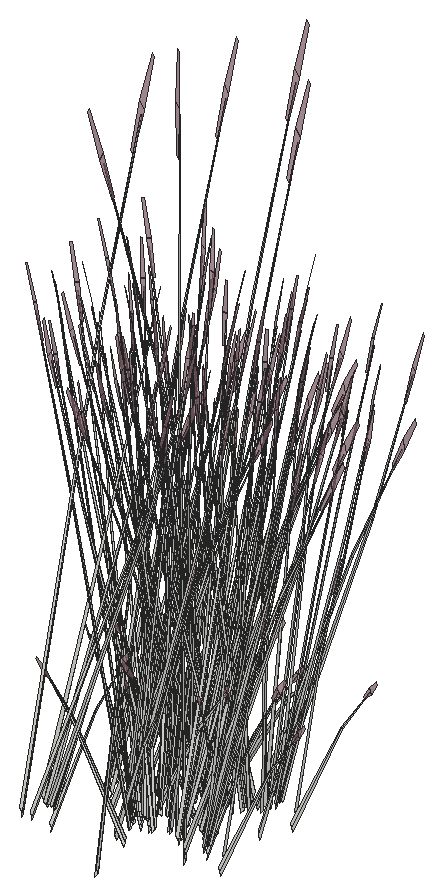
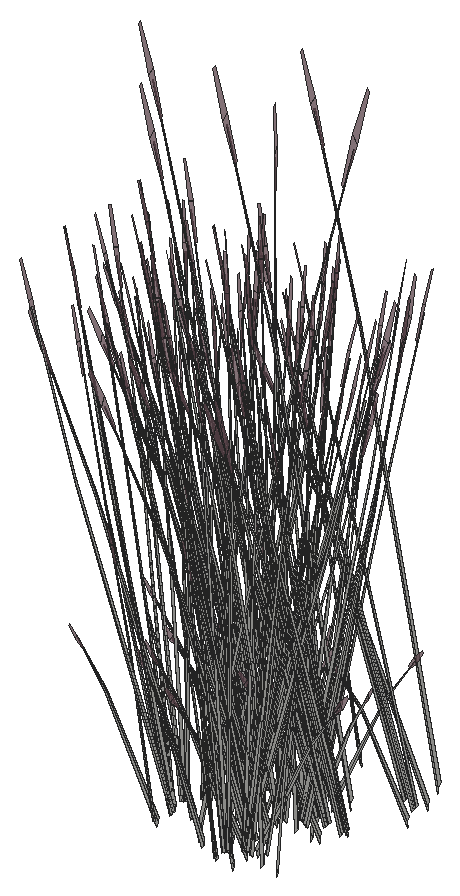
# SketchUp Ruby script. Lengths in inches.
U = 1.inch
M = Sketchup.active_model
def pt(a) = Geom::Point3d.new(a.map { |v| v * U })
def face(e, loops, mat)
  f = e.add_face(loops[0].map { |a| pt(a) })
  loops[1..].each { |l| e.add_face(l.map { |a| pt(a) }).erase! }
  f.material = f.back_material = mat if mat
  f
end
# faces: each face lists its corners as indices into pts; further lists are holes
def faces(e, pts, list, mat = nil) = list.each { |f| face(e, (f[0].is_a?(Array) ? f : [f]).map { |l| l.map { |i| pts[i] } }, mat) }
# xy, xz, yz: faces in a plane at the given z, y or x. An outline is a flat list of corners, or four numbers for a rectangle; further outlines are holes
def ring(l) = l.size == 4 ? [[l[0], l[1]], [l[2], l[1]], [l[2], l[3]], [l[0], l[3]]] : l.each_slice(2).to_a
def flat(e, list, mat, &to3) = list.each { |f| face(e, (f[0].is_a?(Array) ? f : [f]).map { |l| ring(l).map { |u, v| to3.(u, v) } }, mat) }
def xy(e, z, list, mat = nil) = flat(e, list, mat) { |x, y| [x, y, z] }
def xz(e, y, list, mat = nil) = flat(e, list, mat) { |x, z| [x, y, z] }
def yz(e, x, list, mat = nil) = flat(e, list, mat) { |y, z| [x, y, z] }
def lines(e, pts, list) = list.each { |a, b| e.add_line(pt(pts[a]), pt(pts[b])) }
# prism: a flat outline (further loops are holes) pulled along v
def prism(e, loops, v, mat = nil)
  f = face(e, loops, mat); d = Geom::Vector3d.new(v.map { |x| x * U })
  f.pushpull(f.normal.samedirection?(d) ? d.length : -d.length)
end
def box(e, o, s, mat = nil) = prism(e, [[o, [o[0] + s[0], o[1], o[2]], [o[0] + s[0], o[1] + s[1], o[2]], [o[0], o[1] + s[1], o[2]]]], [0, 0, s[2]], mat)
def at(x, y, z, deg = 0) = Geom::Transformation.translation(pt([x, y, z])) * Geom::Transformation.rotation(ORIGIN, Z_AXIS, deg.degrees)
def axes(o, x, y, z) = Geom::Transformation.new([*x, 0, *y, 0, *z, 0, *pt(o).to_a, 1])
def part(name) = M.definitions.add(name)
# library, detail: a bought-in or finely detailed component or shape, given as its bounding box
def library(name, o, s) = part(name).tap { |d| box(d.entities, o, s) }
def detail(e, o, s) = box(e.add_group.entities, o, s)
def put(e, d, t, mat = nil) = e.add_instance(d, t).tap { |i| i.material = mat if mat }
def group(e, t, mat = nil) = e.add_group.tap { |g| g.transformation = t; g.material = mat if mat }.entities
root = M.entities
M.materials.add("LightPink_Translucent").color = [144, 107, 117]
M.materials["LightPink_Translucent"].alpha = 0.75
c1 = part("blade")
p = [[2.15,0.21,22],[0,0.17,0],[0.09,0.45,0],[2.18,0.31,22],[2.29,0.31,22],[0.38,0.45,0],
  [2.48,0.24,33],[2.49,0.24,33],[2.48,0.22,33]]
faces(c1.entities,p,[[0,1,2,3],[4,5,2,3],[6,3,4,7],[8,0,3,6]])
c2 = part("seeds")
p = [[0.3,-0.1,1.38],[-0.01,-0.03,1.59],[-0.01,-0.03,0.03],[0.14,-0.07,-0.07],[0.29,-0.03,3],[0.15,0.01,3.11]]
faces(c2.entities,p,[[0,1,2,3],[1,0,4,5]],"LightPink_Translucent")
c3 = part("blade with seeds")
put(c3.entities,c1,at(0,0,0))
put(c3.entities,c2,axes([2.4,0.25,30.99],[1.5799,-0.05474,1.17369],[-0.12525,1.92788,0.29478],[-0.07173,-0.02425,1.56792]))
put(root,c3,axes([337.16,22.48,50.44],[0.32236,-0.02796,1.01491],[-0.20448,0.24636,0.74569],[-0.1593,-0.03696,0.22354]))
put(root,c3,axes([333,21.07,52.4],[0.50473,0.00941,-0.62776],[-0.0339,0.39618,0.07576],[0.21383,0.04181,0.88802]))
put(root,c3,axes([336.36,22.91,50.44],[-0.16818,0.19891,1.01491],[-0.14456,-0.26725,0.74569],[0.1389,-0.06697,0.22354]))
put(root,c3,axes([338.18,21.87,52.45],[-0.02704,0.39739,-0.10745],[-0.51189,-0.01086,-0.59638],[-0.19715,-0.0276,0.90619]))
put(root,c3,axes([342.01,23.39,52.45],[-0.25405,-0.35383,-0.10745],[0.45089,-0.17388,-0.59638],[0.19001,-0.04668,0.90619]))
put(root,c3,axes([341.98,23.09,52.14],[0.13679,-0.35544,-0.45151],[0.46898,0.12183,-0.34973],[0.18882,-0.03259,0.86392]))
put(root,c3,axes([338.31,18.42,50.97],[0.01109,-0.20172,1.3638],[0.49896,0.10655,0.18846],[-0.04323,0.21498,0.64398]))
put(root,c3,axes([336.12,23.66,52],[0.43951,-0.05584,-0.31292],[0.11606,0.31924,0.40398],[0.12595,-0.08575,0.77298]))
put(root,c3,axes([333.31,21.23,52],[0.28729,0.24465,-0.31292],[-0.32804,0.23159,0.40398],[0.16667,0.03524,0.77298]))
put(root,c3,axes([341.9,23.22,52.4],[0.44368,-0.17257,-0.62776],[0.24726,0.35524,0.07576],[0.21437,-0.04035,0.88802]))
put(root,c3,axes([332.28,20.6,51.43],[-0.18755,-0.06732,1.51428],[0.38813,-0.28243,0.12244],[0.24191,0.12741,0.64734]))
put(root,c3,axes([332.3125,19.72,51.95],[-0.4363,-0.20303,1.22187],[0.46069,-0.31611,0.5272],[0.14077,0.1905,1.18105]))
put(root,c3,axes([332.97,21.37,50.44],[-0.28429,-0.11236,1.01491],[0.36709,-0.11416,0.74569],[0.09901,0.0967,0.22354]))
put(root,c3,axes([342.27,23.25,52],[0.41962,0.10901,-0.31292],[-0.12239,0.31802,0.40398],[0.16894,-0.02916,0.77298]))
put(root,c3,axes([331.97,21.69,52.45],[0.30087,-0.33447,-0.10745],[0.43572,0.19269,-0.59638],[0.15146,0.0945,0.90619]))
put(root,c3,axes([341.13,22.86,51.43],[-0.20943,0.00885,1.51428],[0.13893,-0.38357,0.12244],[0.29846,0.02372,0.64734]))
put(root,c3,axes([332.33,21.52,52.14],[0.49824,-0.09289,-0.45151],[0.08716,0.35177,-0.34973],[0.13382,0.10081,0.86392]))
put(root,c3,axes([335.96,26.6,52.4],[-0.24099,-0.31773,-0.62776],[0.49607,-0.17707,0.07576],[-0.05635,-0.15352,0.88802]))
put(root,c3,axes([336.01,24.72,52.45],[-0.25405,-0.35383,-0.10745],[0.45089,-0.17388,-0.59638],[0.19001,-0.04668,0.90619]))
put(root,c3,axes([335.98,24.42,52.14],[0.13679,-0.35544,-0.45151],[0.46898,0.12183,-0.34973],[0.18882,-0.03259,0.86392]))
put(root,c3,axes([336.96,26.91,52.4],[0.01314,-0.36145,-0.62776],[0.55324,0.02428,0.07576],[0.05838,-0.15313,0.88802]))
put(root,c3,axes([335.9,24.55,52.4],[0.44368,-0.17257,-0.62776],[0.24726,0.35524,0.07576],[0.21437,-0.04035,0.88802]))
put(root,c3,axes([343.16,23.32,50.44],[-0.31197,0.06451,1.01491],[0.14684,-0.26661,0.74569],[0.1655,0.01824,0.22354]))
put(root,c3,axes([336,26.33,52],[0.15222,-0.30049,-0.31292],[0.44409,0.08764,0.40398],[-0.04072,-0.12098,0.77298]))
put(root,c3,axes([336.34,26.73,51.43],[-0.09401,0.13431,1.51428],[-0.3944,-0.27795,0.12244],[0.17792,-0.17323,0.64734]))
put(root,c3,axes([335.78,26.54,52.14],[-0.49634,-0.09796,-0.45151],[0.17013,-0.33585,-0.34973],[-0.04551,-0.13522,0.86392]))
put(root,c3,axes([336.08,25.7,50.44],[0.06477,0.22786,1.01491],[-0.35932,-0.1262,0.74569],[0.03867,-0.11667,0.22354]))
put(root,c3,axes([336.85,26.79,52.14],[-0.36145,-0.26255,-0.45151],[0.38183,-0.22994,-0.34973],[0.055,-0.1334,0.86392]))
put(root,c3,axes([337.63,22.91,52.14],[-0.13679,0.35544,-0.45151],[-0.46898,-0.12183,-0.34973],[-0.18882,0.03259,0.86392]))
put(root,c3,axes([337.61,22.6,52.45],[0.25405,0.35383,-0.10745],[-0.45089,0.17388,-0.59638],[-0.19001,0.04668,0.90619]))
put(root,c3,axes([342.62,24.14,51.47],[-0.09664,-0.32847,-0.03085],[0.45676,-0.07551,-0.13989],[0.09538,0.02082,0.4614]))
put(root,c3,axes([341.4375,24.13,52.45],[0.02704,-0.39739,-0.10745],[0.51189,0.01086,-0.59638],[0.19715,0.0276,0.90619]))
put(root,c3,axes([338.69,27.6,51.43],[0.11542,0.12546,1.51428],[-0.53333,0.10562,0.12244],[-0.12054,-0.19696,0.64734]))
put(root,c3,axes([336.2,26.52,52.45],[-0.49409,0.18193,-0.10745],[-0.24281,-0.32289,-0.59638],[-0.06519,-0.13607,0.90619]))
put(root,c3,axes([337.23,26.93,52.45],[-0.55492,-0.01936,-0.10745],[0.01517,-0.36657,-0.59638],[0.03855,-0.14118,0.90619]))
put(root,c3,axes([336.27,24.58,52],[0.41962,0.10901,-0.31292],[-0.12239,0.31802,0.40398],[0.16894,-0.02916,0.77298]))
put(root,c3,axes([337.19,26.69,52],[0.34164,-0.20573,-0.31292],[0.3234,0.23491,0.40398],[0.04921,-0.11936,0.77298]))
put(root,c3,axes([340.11,27.69,52.4],[-0.24099,-0.31773,-0.62776],[0.49607,-0.17707,0.07576],[-0.05635,-0.15352,0.88802]))
put(root,c3,axes([335.13,24.18,51.43],[-0.20943,0.00885,1.51428],[0.13893,-0.38357,0.12244],[0.29846,0.02372,0.64734]))
put(root,c3,axes([341.12,28.01,52.4],[0.01314,-0.36145,-0.62776],[0.55324,0.02428,0.07576],[0.05838,-0.15313,0.88802]))
put(root,c3,axes([341.46,23.9375,52.4],[0.50473,0.00941,-0.62776],[-0.0339,0.39618,0.07576],[0.21383,0.04181,0.88802]))
put(root,c3,axes([340.16,27.42,52],[0.15222,-0.30049,-0.31292],[0.44409,0.08764,0.40398],[-0.04072,-0.12098,0.77298]))
put(root,c3,axes([340.5,27.82,51.43],[-0.09401,0.13431,1.51428],[-0.3944,-0.27795,0.12244],[0.17792,-0.17323,0.64734]))
put(root,c3,axes([339.93,27.63,52.14],[-0.49634,-0.09796,-0.45151],[0.17013,-0.33585,-0.34973],[-0.04551,-0.13522,0.86392]))
put(root,c3,axes([340.24,26.79,50.44],[0.06477,0.22786,1.01491],[-0.35932,-0.1262,0.74569],[0.03867,-0.11667,0.22354]))
put(root,c3,axes([337.16,24.64,50.44],[-0.31197,0.06451,1.01491],[0.14684,-0.26661,0.74569],[0.1655,0.01824,0.22354]))
put(root,c3,axes([341.01,27.89,52.14],[-0.36145,-0.26255,-0.45151],[0.38183,-0.22994,-0.34973],[0.055,-0.1334,0.86392]))
put(root,c3,axes([337.61,27.54,52.4],[0.26374,-0.30832,-0.62776],[0.46217,0.21911,0.07576],[0.15748,-0.11171,0.88802]))
put(root,c3,axes([337.6,27.4,52.14],[-0.12971,-0.3568,-0.45151],[0.49122,-0.06241,-0.34973],[0.14077,-0.09583,0.86392]))
put(root,c3,axes([336.7,24.43,50.44],[0.21042,-0.1771,1.01491],[0.08303,0.28036,0.74569],[-0.15207,0.0502,0.22354]))
put(root,c3,axes([341.77,24.1,52],[0.28729,0.24465,-0.31292],[-0.32804,0.23159,0.40398],[0.16667,0.03524,0.77298]))
put(root,c3,axes([337.49,23.66,52],[-0.43951,0.05584,-0.31292],[-0.11606,-0.31924,0.40398],[-0.12595,0.08575,0.77298]))
put(root,c3,axes([337.83,27.65,52.45],[-0.46706,-0.21546,-0.10745],[0.26908,-0.31203,-0.59638],[0.13196,-0.10846,0.90619]))
put(root,c3,axes([340.36,27.61,52.45],[-0.49409,0.18193,-0.10745],[-0.24281,-0.32289,-0.59638],[-0.06519,-0.13607,0.90619]))
put(root,c3,axes([336.62,25.46,51.47],[-0.09664,-0.32847,-0.03085],[0.45676,-0.07551,-0.13989],[0.09538,0.02082,0.4614]))
put(root,c3,axes([341.38,28.02,52.45],[-0.55492,-0.01936,-0.10745],[0.01517,-0.36657,-0.59638],[0.03855,-0.14118,0.90619]))
put(root,c3,axes([341.35,27.79,52],[0.34164,-0.20573,-0.31292],[0.3234,0.23491,0.40398],[0.04921,-0.11936,0.77298]))
put(root,c3,axes([335.4375,25.45,52.45],[0.02704,-0.39739,-0.10745],[0.51189,0.01086,-0.59638],[0.19715,0.0276,0.90619]))
put(root,c3,axes([338.39,27.0625,50.44],[0.26338,0.136,1.01491],[-0.38358,0.08175,0.74569],[-0.08207,-0.10452,0.22354]))
put(root,c3,axes([339.03,27.78,52.4],[-0.43054,-0.18887,-0.62776],[0.30598,-0.33097,0.07576],[-0.15599,-0.11277,0.88802]))
put(root,c3,axes([338.88,27.53,52],[-0.07798,-0.31474,-0.31292],[0.44579,-0.08311,0.40398],[-0.11974,-0.09019,0.77298]))
put(root,c3,axes([340.73,23.47,51.43],[-0.18755,-0.06732,1.51428],[0.38813,-0.28243,0.12244],[0.24191,0.12741,0.64734]))
put(root,c3,axes([340.77,22.59,51.95],[-0.4363,-0.20303,1.22187],[0.46069,-0.31611,0.5272],[0.14077,0.1905,1.18105]))
put(root,c3,axes([338.2,26.6875,50.44],[-0.16818,0.19891,1.01491],[-0.14456,-0.26725,0.74569],[0.1389,-0.06697,0.22354]))
put(root,c3,axes([337.625,23.44,52.45],[0.46706,0.21546,-0.10745],[-0.26908,0.31203,-0.59638],[-0.13196,0.10846,0.90619]))
put(root,c3,axes([341.43,24.24,50.44],[-0.28429,-0.11236,1.01491],[0.36709,-0.11416,0.74569],[0.09901,0.0967,0.22354]))
put(root,c3,axes([340.43,24.5625,52.45],[0.30087,-0.33447,-0.10745],[0.43572,0.19269,-0.59638],[0.15146,0.0945,0.90619]))
put(root,c3,axes([337.96,27.43,52],[0.43951,-0.05584,-0.31292],[0.11606,0.31924,0.40398],[0.12595,-0.08575,0.77298]))
put(root,c3,axes([338.25,23.35,51.43],[0.12611,-0.12006,1.51428],[0.31843,0.32408,0.12244],[-0.2184,0.14759,0.64734]))
put(root,c3,axes([337.86,23.7,52.14],[0.12971,0.3568,-0.45151],[-0.49122,0.06241,-0.34973],[-0.14077,0.09583,0.86392]))
put(root,c3,axes([338.83,27.79,52.14],[-0.49824,0.09289,-0.45151],[-0.08716,-0.35177,-0.34973],[-0.13382,-0.10081,0.86392]))
put(root,c3,axes([340.74,22.98,50.51],[-0.01379,-0.36791,1.24828],[0.62424,0.09537,0.52853],[-0.14764,0.20132,1.17828]))
put(root,c3,axes([335.46,25.26,52.4],[0.50473,0.00941,-0.62776],[-0.0339,0.39618,0.07576],[0.21383,0.04181,0.88802]))
put(root,c3,axes([340.79,24.4,52.14],[0.49824,-0.09289,-0.45151],[0.08716,0.35177,-0.34973],[0.13382,0.10081,0.86392]))
put(root,c3,axes([341.77,28.63,52.4],[0.26374,-0.30832,-0.62776],[0.46217,0.21911,0.07576],[0.15748,-0.11171,0.88802]))
put(root,c3,axes([341.76,28.49,52.14],[-0.12971,-0.3568,-0.45151],[0.49122,-0.06241,-0.34973],[0.14077,-0.09583,0.86392]))
put(root,c3,axes([341.99,28.75,52.45],[-0.46706,-0.21546,-0.10745],[0.26908,-0.31203,-0.59638],[0.13196,-0.10846,0.90619]))
put(root,c3,axes([335.77,25.43,52],[0.28729,0.24465,-0.31292],[-0.32804,0.23159,0.40398],[0.16667,0.03524,0.77298]))
put(root,c3,axes([340.06,29.92,50.9375],[0.43633,0.15757,1.33654],[-0.42745,0.33945,0.52853],[-0.19146,-0.20119,1.12046]))
put(root,c3,axes([338.16,23.64,51.43],[0.09401,-0.13431,1.51428],[0.3944,0.27795,0.12244],[-0.17792,0.17323,0.64734]))
put(root,c3,axes([342.36,27.78,50.44],[-0.16818,0.19891,1.01491],[-0.14456,-0.26725,0.74569],[0.1389,-0.06697,0.22354]))
put(root,c3,axes([338.27,24.4,52],[-0.34164,0.20573,-0.31292],[-0.3234,-0.23491,0.40398],[-0.04921,0.11936,0.77298]))
put(root,c3,axes([339.25,24.57,52.45],[0.49409,-0.18193,-0.10745],[0.24281,0.32289,-0.59638],[0.06519,0.13607,0.90619]))
put(root,c3,axes([338.48,25.2,50.44],[-0.01307,-0.23234,1.01491],[0.32652,0.16572,0.74569],[-0.06422,0.11074,0.22354]))
put(root,c3,axes([334.73,24.8,51.43],[-0.18755,-0.06732,1.51428],[0.38813,-0.28243,0.12244],[0.24191,0.12741,0.64734]))
put(root,c3,axes([342.12,28.53,52],[0.43951,-0.05584,-0.31292],[0.11606,0.31924,0.40398],[0.12595,-0.08575,0.77298]))
put(root,c3,axes([334.77,23.91,51.95],[-0.4363,-0.20303,1.22187],[0.46069,-0.31611,0.5272],[0.14077,0.1905,1.18105]))
put(root,c3,axes([337.85,28.09,52],[-0.28729,-0.24465,-0.31292],[0.32804,-0.23159,0.40398],[-0.16667,-0.03524,0.77298]))
put(root,c3,axes([337.85,28.49,52.45],[-0.25405,-0.35383,-0.10745],[0.45089,-0.17388,-0.59638],[0.19001,-0.04668,0.90619]))
put(root,c3,axes([337.83,28.1875,52.14],[0.13679,-0.35544,-0.45151],[0.46898,0.12183,-0.34973],[0.18882,-0.03259,0.86392]))
put(root,c3,axes([335.43,25.57,50.44],[-0.28429,-0.11236,1.01491],[0.36709,-0.11416,0.74569],[0.09901,0.0967,0.22354]))
put(root,c3,axes([338.61,24.3,52.42],[0.36145,0.26255,-0.50118],[-0.38183,0.22994,-0.3882],[-0.055,0.1334,0.95895]))
put(root,c3,axes([334.43,25.89,52.45],[0.30087,-0.33447,-0.10745],[0.43572,0.19269,-0.59638],[0.15146,0.0945,0.90619]))
put(root,c3,axes([339.68,24.56,52.14],[0.49634,0.09796,-0.45151],[-0.17013,0.33585,-0.34973],[0.04551,0.13522,0.86392]))
put(root,c3,axes([339.96,23.87,51.43],[-0.11542,-0.12546,1.51428],[0.53333,-0.10562,0.12244],[0.12054,0.19696,0.64734]))
put(root,c3,axes([339.45,24.76,52],[-0.15222,0.30049,-0.31292],[-0.44409,-0.08764,0.40398],[0.04072,0.12098,0.77298]))
put(root,c3,axes([337.74,28.32,52.4],[0.44368,-0.17257,-0.62776],[0.24726,0.35524,0.07576],[0.21437,-0.04035,0.88802]))
put(root,c3,axes([338.49,24.18,52.72],[-0.01314,0.36145,-0.69681],[-0.55324,-0.02428,0.08409],[-0.05838,0.15313,0.9857]))
put(root,c3,axes([334.79,25.72,52.14],[0.49824,-0.09289,-0.45151],[0.08716,0.35177,-0.34973],[0.13382,0.10081,0.86392]))
put(root,c3,axes([336.05,30.88,52.4],[0.01314,-0.36145,-0.62776],[0.55324,0.02428,0.07576],[0.05838,-0.15313,0.88802]))
put(root,c3,axes([339.02,23.93,51.43],[-0.01236,-0.14998,1.51428],[0.53562,0.09949,0.12244],[-0.03313,0.21373,0.64734]))
put(root,c3,axes([336.82,30.32,52.17],[-0.00487,-0.07777,1.54581],[-0.41166,-0.22476,-0.24447],[0.06364,-0.13625,0.12397]))
put(root,c3,axes([335.09,30.3,52],[0.15222,-0.30049,-0.31292],[0.44409,0.08764,0.40398],[-0.04072,-0.12098,0.77298]))
put(root,c3,axes([335.43,30.7,51.43],[-0.09401,0.13431,1.51428],[-0.3944,-0.27795,0.12244],[0.17792,-0.17323,0.64734]))
put(root,c3,axes([339.5,24.49,52.4],[0.24099,0.31773,-0.62776],[-0.49607,0.17707,0.07576],[0.05635,0.15352,0.88802]))
put(root,c3,axes([335.17,29.67,50.44],[0.06477,0.22786,1.01491],[-0.35932,-0.1262,0.74569],[0.03867,-0.11667,0.22354]))
put(root,c3,axes([335.94,30.76,52.14],[-0.36145,-0.26255,-0.45151],[0.38183,-0.22994,-0.34973],[0.055,-0.1334,0.86392]))
put(root,c3,axes([337.98,28.33,52.14],[-0.36663,0.25884,-0.45151],[-0.32109,-0.27343,-0.34973],[-0.18628,-0.03938,0.86392]))
put(root,c3,axes([337.16,28.67,50.44],[0.32236,-0.02796,1.01491],[-0.20448,0.24636,0.74569],[-0.1593,-0.03696,0.22354]))
put(root,c3,axes([338.12,28.35,52],[0.41962,0.10901,-0.31292],[-0.12239,0.31802,0.40398],[0.16894,-0.02916,0.77298]))
put(root,c3,axes([338.18,28.0625,52.45],[-0.02704,0.39739,-0.10745],[-0.51189,-0.01086,-0.59638],[-0.19715,-0.0276,0.90619]))
put(root,c3,axes([333.25,25.9,52.45],[0.49409,-0.18193,-0.10745],[0.24281,0.32289,-0.59638],[0.06519,0.13607,0.90619]))
put(root,c3,axes([342.01,29.59,52.45],[-0.25405,-0.35383,-0.10745],[0.45089,-0.17388,-0.59638],[0.19001,-0.04668,0.90619]))
put(root,c3,axes([341.98,29.28,52.14],[0.13679,-0.35544,-0.45151],[0.46898,0.12183,-0.34973],[0.18882,-0.03259,0.86392]))
put(root,c3,axes([336.32,30.9,52.45],[-0.55492,-0.01936,-0.10745],[0.01517,-0.36657,-0.59638],[0.03855,-0.14118,0.90619]))
put(root,c3,axes([336.28,30.67,52],[0.34164,-0.20573,-0.31292],[0.3234,0.23491,0.40398],[0.04921,-0.11936,0.77298]))
put(root,c3,axes([338.31,24.69,50.97],[0.01109,-0.20172,1.3638],[0.49896,0.10655,0.18846],[-0.04323,0.21498,0.64398]))
put(root,c3,axes([336.97,27.96,51.43],[-0.20943,0.00885,1.51428],[0.13893,-0.38357,0.12244],[0.29846,0.02372,0.64734]))
put(root,c3,axes([341.9,29.41,52.4],[0.44368,-0.17257,-0.62776],[0.24726,0.35524,0.07576],[0.21437,-0.04035,0.88802]))
put(root,c3,axes([333.68,25.88,52.14],[0.49634,0.09796,-0.45151],[-0.17013,0.33585,-0.34973],[0.04551,0.13522,0.86392]))
put(root,c3,axes([333.96,25.19,51.43],[-0.11542,-0.12546,1.51428],[0.53333,-0.10562,0.12244],[0.12054,0.19696,0.64734]))
put(root,c3,axes([333.45,26.09,52],[-0.15222,0.30049,-0.31292],[-0.44409,-0.08764,0.40398],[0.04072,0.12098,0.77298]))
put(root,c3,axes([339.01,28.41,50.44],[-0.31197,0.06451,1.01491],[0.14684,-0.26661,0.74569],[0.1655,0.01824,0.22354]))
put(root,c3,axes([336.7,31.51,52.4],[0.26374,-0.30832,-0.62776],[0.46217,0.21911,0.07576],[0.15748,-0.11171,0.88802]))
put(root,c3,axes([333.5,25.82,52.4],[0.24099,0.31773,-0.62776],[-0.49607,0.17707,0.07576],[0.05635,0.15352,0.88802]))
put(root,c3,axes([336.69,31.37,52.14],[-0.12971,-0.3568,-0.45151],[0.49122,-0.06241,-0.34973],[0.14077,-0.09583,0.86392]))
put(root,c3,axes([338.46,29.24,51.47],[-0.09664,-0.32847,-0.03085],[0.45676,-0.07551,-0.13989],[0.09538,0.02082,0.4614]))
put(root,c3,axes([342.27,29.44,52],[0.41962,0.10901,-0.31292],[-0.12239,0.31802,0.40398],[0.16894,-0.02916,0.77298]))
put(root,c3,axes([337.28,29.23,52.45],[0.02704,-0.39739,-0.10745],[0.51189,0.01086,-0.59638],[0.19715,0.0276,0.90619]))
put(root,c3,axes([336.92,31.625,52.45],[-0.46706,-0.21546,-0.10745],[0.26908,-0.31203,-0.59638],[0.13196,-0.10846,0.90619]))
put(root,c3,axes([341.13,29.05,51.43],[-0.20943,0.00885,1.51428],[0.13893,-0.38357,0.12244],[0.29846,0.02372,0.64734]))
put(root,c3,axes([337.29,30.66,50.44],[-0.16818,0.19891,1.01491],[-0.14456,-0.26725,0.74569],[0.1389,-0.06697,0.22354]))
put(root,c3,axes([337.05,31.41,52],[0.43951,-0.05584,-0.31292],[0.11606,0.31924,0.40398],[0.12595,-0.08575,0.77298]))
put(root,c3,axes([343.16,29.51,50.44],[-0.31197,0.06451,1.01491],[0.14684,-0.26661,0.74569],[0.1655,0.01824,0.22354]))
put(root,c3,axes([337.31,29.04,52.4],[0.50473,0.00941,-0.62776],[-0.0339,0.39618,0.07576],[0.21383,0.04181,0.88802]))
put(root,c3,axes([337.63,29.1,52.14],[-0.13679,0.35544,-0.45151],[-0.46898,-0.12183,-0.34973],[-0.18882,0.03259,0.86392]))
put(root,c3,axes([337.61,28.8,52.45],[0.25405,0.35383,-0.10745],[-0.45089,0.17388,-0.59638],[-0.19001,0.04668,0.90619]))
put(root,c3,axes([342.62,30.33,51.47],[-0.09664,-0.32847,-0.03085],[0.45676,-0.07551,-0.13989],[0.09538,0.02082,0.4614]))
put(root,c3,axes([337.61,29.2,52],[0.28729,0.24465,-0.31292],[-0.32804,0.23159,0.40398],[0.16667,0.03524,0.77298]))
put(root,c3,axes([341.4375,30.32,52.45],[0.02704,-0.39739,-0.10745],[0.51189,0.01086,-0.59638],[0.19715,0.0276,0.90619]))
put(root,c3,axes([338.32,31.91,52.17],[0.07006,-0.05952,1.54581],[-0.08968,-0.3651,-0.24447],[0.1758,-0.06922,0.12397]))
put(root,c3,axes([336.58,28.57,51.43],[-0.18755,-0.06732,1.51428],[0.38813,-0.28243,0.12244],[0.24191,0.12741,0.64734]))
put(root,c3,axes([336.61,27.6875,51.95],[-0.4363,-0.20303,1.22187],[0.46069,-0.31611,0.5272],[0.14077,0.1905,1.18105]))
put(root,c3,axes([337.27,29.34,50.44],[-0.28429,-0.11236,1.01491],[0.36709,-0.11416,0.74569],[0.09901,0.0967,0.22354]))
put(root,c3,axes([336.27,29.66,52.45],[0.30087,-0.33447,-0.10745],[0.43572,0.19269,-0.59638],[0.15146,0.0945,0.90619]))
put(root,c3,axes([341.46,30.13,52.4],[0.50473,0.00941,-0.62776],[-0.0339,0.39618,0.07576],[0.21383,0.04181,0.88802]))
put(root,c3,axes([336.94,32.46,52.45],[-0.25405,-0.35383,-0.10745],[0.45089,-0.17388,-0.59638],[0.19001,-0.04668,0.90619]))
put(root,c3,axes([336.92,32.16,52.14],[0.13679,-0.35544,-0.45151],[0.46898,0.12183,-0.34973],[0.18882,-0.03259,0.86392]))
